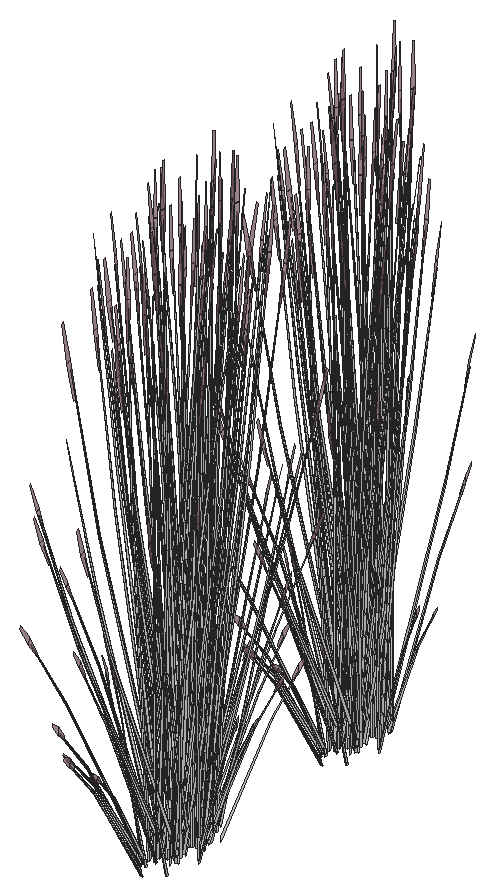
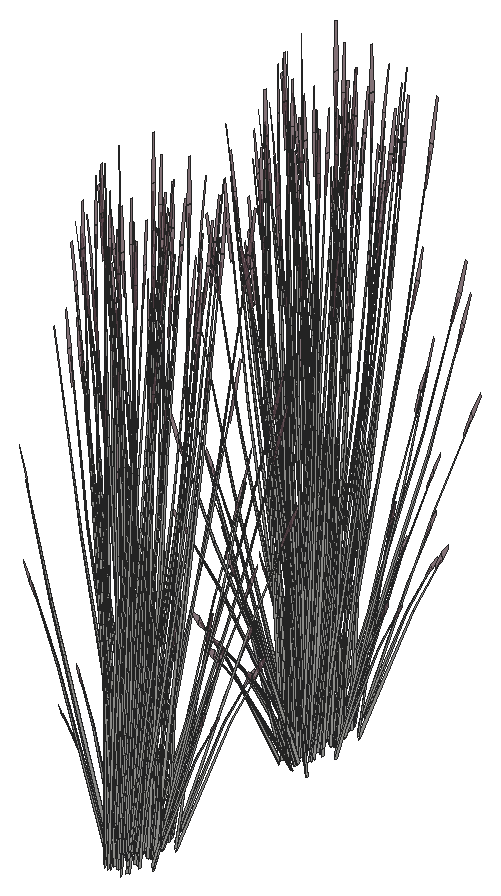
# SketchUp Ruby script. Lengths in inches.
U = 1.inch
M = Sketchup.active_model
def pt(a) = Geom::Point3d.new(a.map { |v| v * U })
def face(e, loops, mat)
  f = e.add_face(loops[0].map { |a| pt(a) })
  loops[1..].each { |l| e.add_face(l.map { |a| pt(a) }).erase! }
  f.material = f.back_material = mat if mat
  f
end
# faces: each face lists its corners as indices into pts; further lists are holes
def faces(e, pts, list, mat = nil) = list.each { |f| face(e, (f[0].is_a?(Array) ? f : [f]).map { |l| l.map { |i| pts[i] } }, mat) }
# xy, xz, yz: faces in a plane at the given z, y or x. An outline is a flat list of corners, or four numbers for a rectangle; further outlines are holes
def ring(l) = l.size == 4 ? [[l[0], l[1]], [l[2], l[1]], [l[2], l[3]], [l[0], l[3]]] : l.each_slice(2).to_a
def flat(e, list, mat, &to3) = list.each { |f| face(e, (f[0].is_a?(Array) ? f : [f]).map { |l| ring(l).map { |u, v| to3.(u, v) } }, mat) }
def xy(e, z, list, mat = nil) = flat(e, list, mat) { |x, y| [x, y, z] }
def xz(e, y, list, mat = nil) = flat(e, list, mat) { |x, z| [x, y, z] }
def yz(e, x, list, mat = nil) = flat(e, list, mat) { |y, z| [x, y, z] }
def lines(e, pts, list) = list.each { |a, b| e.add_line(pt(pts[a]), pt(pts[b])) }
# prism: a flat outline (further loops are holes) pulled along v
def prism(e, loops, v, mat = nil)
  f = face(e, loops, mat); d = Geom::Vector3d.new(v.map { |x| x * U })
  f.pushpull(f.normal.samedirection?(d) ? d.length : -d.length)
end
def box(e, o, s, mat = nil) = prism(e, [[o, [o[0] + s[0], o[1], o[2]], [o[0] + s[0], o[1] + s[1], o[2]], [o[0], o[1] + s[1], o[2]]]], [0, 0, s[2]], mat)
def at(x, y, z, deg = 0) = Geom::Transformation.translation(pt([x, y, z])) * Geom::Transformation.rotation(ORIGIN, Z_AXIS, deg.degrees)
def axes(o, x, y, z) = Geom::Transformation.new([*x, 0, *y, 0, *z, 0, *pt(o).to_a, 1])
def part(name) = M.definitions.add(name)
# library, detail: a bought-in or finely detailed component or shape, given as its bounding box
def library(name, o, s) = part(name).tap { |d| box(d.entities, o, s) }
def detail(e, o, s) = box(e.add_group.entities, o, s)
def put(e, d, t, mat = nil) = e.add_instance(d, t).tap { |i| i.material = mat if mat }
def group(e, t, mat = nil) = e.add_group.tap { |g| g.transformation = t; g.material = mat if mat }.entities
root = M.entities
M.materials.add("LightPink_Translucent").color = [144, 107, 117]
M.materials["LightPink_Translucent"].alpha = 0.75
c1 = part("blade")
p = [[2.15,0.21,22],[0,0.17,0],[0.09,0.45,0],[2.18,0.31,22],[2.29,0.31,22],[0.38,0.45,0],
  [2.48,0.24,33],[2.49,0.24,33],[2.48,0.22,33]]
faces(c1.entities,p,[[0,1,2,3],[4,5,2,3],[6,3,4,7],[8,0,3,6]])
c2 = part("seeds")
p = [[0.3,-0.1,1.38],[-0.01,-0.03,1.59],[-0.01,-0.03,0.03],[0.14,-0.07,-0.07],[0.29,-0.03,3],[0.15,0.01,3.11]]
faces(c2.entities,p,[[0,1,2,3],[1,0,4,5]],"LightPink_Translucent")
c3 = part("blade with seeds")
put(c3.entities,c1,at(0,0,0))
put(c3.entities,c2,axes([2.4,0.25,30.99],[1.5799,-0.05474,1.17369],[-0.12525,1.92788,0.29478],[-0.07173,-0.02425,1.56792]))
put(root,c3,axes([252.15,10.32,1.07],[-0.07276,0.12376,1.03788],[-0.21789,-0.21662,-0.22321],[0.04039,-0.2694,0.44375]))
put(root,c3,axes([251.82,10.75,2.81],[-0.12216,-0.49718,-0.51563],[0.25147,-0.27708,0.06223],[-0.02857,-0.24022,0.72942]))
put(root,c3,axes([251.03,10.09,1.07],[-0.0155,0.20002,1.03788],[-0.22659,0.16744,-0.22321],[-0.05297,-0.25854,0.44375]))
put(root,c3,axes([251.61,9.65,0.28],[-0.04293,0.02203,1.27986],[-0.23742,-0.24798,-0.19552],[0.00398,-0.20684,0.218]))
put(root,c3,axes([252.33,11.24,2.81],[0.00666,-0.56559,-0.51563],[0.28045,0.03799,0.06223],[0.0296,-0.23961,0.72942]))
put(root,c3,axes([251.88,9.33,1.2],[0.03283,0.35655,0.83364],[-0.18215,-0.19748,0.6125],[0.0196,-0.18257,0.18362]))
put(root,c3,axes([250.95,9.76,1.2],[0.13352,0.21281,0.83364],[-0.19445,0.12793,0.6125],[-0.0416,-0.16355,0.18362]))
put(root,c3,axes([251.27,10.89,2.81],[-0.21825,-0.29555,-0.51563],[0.15511,-0.5179,0.06223],[-0.07907,-0.17646,0.72942]))
put(root,c3,axes([250.84,10.4,0.28],[-0.02479,0.08055,1.27986],[-0.25056,0.17367,-0.19552],[-0.06053,-0.15798,0.218]))
put(root,c3,axes([251.25,12.62,0.72],[-0.10512,-0.62701,-0.50685],[0.30279,-0.22582,-0.13303],[-0.01162,-0.21232,1.11879]))
put(root,c3,axes([252.66,10.7,0.28],[-0.03831,-0.04817,1.27986],[-0.0984,-0.53815,-0.19552],[0.06638,-0.14604,0.218]))
put(root,c3,axes([252.66,12.22,2.81],[0.1337,-0.48245,-0.51563],[0.23429,0.34287,0.06223],[0.07983,-0.1748,0.72942]))
put(root,c3,axes([251.21,10.81,0.91],[-0.16003,-0.61271,0],[0.26773,-0.34169,-0.37456],[0.06098,-0.07782,1.18819]))
put(root,c3,axes([251.56,10.08,0.74],[-0.17688,0.35078,-0.02825],[-0.16207,-0.38418,-0.1281],[-0.01141,-0.10886,0.42251]))
put(root,c3,axes([250.64,12.53,0.66],[0,-0.61145,-0.36036],[0.28637,0,0],[0,-0.13926,1.14313]))
put(root,c3,axes([251.43,10.72,0.66],[0.23955,-0.30573,-0.36036],[0.14318,0.54821,0],[0.05456,-0.06963,1.14313]))
put(root,c3,axes([252.85,11.78,1.07],[-0.09144,-0.01811,1.03788],[-0.09368,-0.48584,-0.22321],[0.11233,-0.13744,0.44375]))
put(root,c3,axes([251.71,11.97,0.6875],[0.1724,-0.45959,-0.45255],[0.21416,0.41674,-0.11877],[0.06908,-0.11465,0.99892]))
put(root,c3,axes([252.96,10.88,1.2],[-0.08525,0.31126,0.83364],[-0.07328,-0.41819,0.6125],[0.07041,-0.10479,0.18362]))
put(root,c3,axes([251.41,12.78,0.8],[0.12419,-0.55096,-0.32471],[0.25804,0.26516,0.15627],[0,-0.12701,1.04254]))
put(root,c3,axes([251.53,12.51,1.13],[-0.02983,-0.6977,-0.21117],[0.31064,-0.04219,-0.36291],[0.0547,-0.09294,1.15913]))
put(root,c3,axes([250.76,12.54,0.66],[0.17867,-0.3815,-0.22483],[0.17867,0.3815,0.22483],[0,-0.12288,1.00865]))
put(root,c3,axes([250.6875,10.71,0.74],[-0.07384,0.49928,-0.02825],[-0.22725,-0.15358,-0.1281],[-0.0345,-0.08166,0.42251]))
put(root,c3,axes([251.38,13.24,1.13],[-0.28825,-0.29175,-0.21117],[0.1388,-0.61578,-0.36291],[-0.00906,-0.15119,1.15913]))
put(root,c3,axes([250.5625,12.99,0.91],[-0.32006,0,0],[0,-0.68339,-0.37456],[0,-0.15565,1.18819]))
put(root,c3,axes([250.62,11.77,1.07],[0.04997,0.17024,1.03788],[-0.11515,0.46273,-0.22321],[-0.11824,-0.1106,0.44375]))
put(root,c3,axes([251.49,10.96,0.66],[0.23879,0.15129,-0.22483],[-0.06012,0.53279,0.22483],[0.04814,-0.06144,1.00865]))
put(root,c3,axes([250.82,11.62,2.81],[-0.25586,-0.01472,-0.51563],[0.01718,-0.61995,0.06223],[-0.1084,-0.06542,0.72942]))
put(root,c3,axes([250.8125,12.8125,0.88],[-0.23808,0.51407,0.22322],[-0.23822,-0.50866,-0.26485],[-0.00831,-0.14599,1.19671]))
put(root,c3,axes([251.57,13.05,0.96],[0.28839,0.29636,0.17466],[-0.1388,0.61578,0.36291],[0,-0.14195,1.16519]))
put(root,c3,axes([251.46,13.89,0.96],[0.06784,-0.72454,-0.17004],[0.32166,0.1263,0.37211],[-0.05621,-0.10006,1.13542]))
put(root,c3,axes([250.32,12.28,1.2],[0.16341,-0.04375,0.83364],[-0.10366,0.38551,0.6125],[-0.08075,-0.05783,0.18362]))
put(root,c3,axes([251.48,12.64,1.17],[-0.27795,0.03775,0.32471],[-0.02514,-0.62656,-0.15627],[0.04976,-0.0635,1.04254]))
put(root,c3,axes([250.76,13.1,0.99],[0,0.61145,0.36036],[-0.28637,0,0],[0,-0.13926,1.14313]))
put(root,c3,axes([252.39,10.97,0.92],[0.16003,-0.61271,0],[0.26773,0.34169,-0.37456],[0.06098,0.07782,1.18819]))
put(root,c3,axes([251.43,13.59,0.8],[-0.15376,-0.51322,-0.32471],[0.2329,-0.3614,0.15627],[-0.04976,-0.0635,1.04254]))
put(root,c3,axes([251.47,12.87,0.91],[0.11128,0.68373,0.33208],[-0.31797,0.23776,0.13031],[0.00389,-0.12563,1.15295]))
put(root,c3,axes([253.02,13.39,0.63],[-0.16485,0.07338,1.02759],[-0.02624,-0.58408,0.05882],[0.11546,-0.08841,0.58473]))
put(root,c3,axes([253.32,12.875,0.83],[-0.15869,-0.39099,-0.04709],[0.1738,-0.35825,-0.21349],[0.04925,-0.02522,0.70419]))
put(root,c3,axes([251.41,13.4,1.17],[-0.12419,0.55096,0.32471],[-0.25804,-0.26516,-0.15627],[0,-0.12701,1.04254]))
put(root,c3,axes([251.87,12.92,0.79],[0,-0.70749,0],[0.32006,0,0],[0,0,1.30246]))
put(root,c3,axes([252.25,11.29,0.99],[-0.23955,-0.30573,0.36036],[0.14318,-0.54821,0],[0.05456,0.06963,1.14313]))
put(root,c3,axes([252.72,13.4375,2.81],[0.22491,-0.27005,-0.51563],[0.12534,0.55588,0.06223],[0.10867,-0.06315,0.72942]))
put(root,c3,axes([251.3,13.79,0.6875],[-0.26625,-0.10025,-0.45255],[0.05619,-0.61836,-0.11877],[-0.07946,-0.07493,0.99892]))
put(root,c3,axes([251.71,12.48,0.91],[-0.21222,0.5549,0.33208],[-0.25213,-0.48983,0.13031],[0.05116,-0.05538,1.15295]))
put(root,c3,axes([251.95,13.47,0.86],[-0.23808,-0.52628,-0.0445],[0.23822,-0.5266,0],[-0.00831,-0.01838,1.27426]))
put(root,c3,axes([251.35,11.56,0.99],[-0.07394,0.60768,0.12804],[-0.27057,-0.17197,0.25465],[0.04674,-0.00296,1.1642]))
put(root,c3,axes([251.23,12.06,0.35],[-0.25194,0.2448,0.93574],[-0.08019,-0.7024,0.36359],[0.1547,0.01169,1.0643]))
put(root,c3,axes([251.91,12.24,1.09],[0.04938,-0.54569,0.10509],[0.24125,0.09472,-0.30009],[0.0439,0.05603,0.91989]))
put(root,c3,axes([251.49,13.54,0.91],[0.32351,0.12883,0.33208],[-0.06584,0.72759,0.13031],[-0.04728,-0.07026,1.15295]))
put(root,c3,axes([253.2,13.01,0.28],[-0.01338,-0.09283,1.27986],[0.09278,-0.54301,-0.19552],[0.09359,-0.00781,0.218]))
put(root,c3,axes([250.44,12.91,0.28],[0.00649,0.09636,1.27986],[-0.13086,0.50324,-0.19552],[-0.09295,-0.02537,0.218]))
put(root,c3,axes([251.81,12.38,1.17],[-0.15376,-0.51322,0.32471],[0.2329,-0.3614,-0.15627],[0.04976,0.0635,1.04254]))
put(root,c3,axes([251.01,14.73,0.66],[-0.06012,-0.53279,-0.22483],[0.23879,-0.15129,0.22483],[-0.04814,-0.06144,1.00865]))
put(root,c3,axes([251.32,14.7,0.99],[0.27504,-0.16229,0.12804],[0.06792,0.60396,0.25465],[-0.02453,-0.088,1.1642]))
put(root,c3,axes([251.89,12.42,1.13],[0.25843,-0.40595,-0.21117],[0.17185,0.5736,-0.36291],[0.06376,0.05825,1.15913]))
put(root,c3,axes([250.95,14.96,0.66],[-0.23955,-0.30573,-0.36036],[0.14318,-0.54821,0],[-0.05456,-0.06963,1.14313]))
put(root,c3,axes([252.54,11.34,0.66],[0.23955,0.30573,-0.36036],[-0.14318,0.54821,0],[0.05456,0.06963,1.14313]))
put(root,c3,axes([252.08,13.08,0.79],[0.28637,0,0],[0,0.63302,0],[0,0,1.29484]))
put(root,c3,axes([251.6,13.88,1.13],[-0.25843,0.40595,-0.21117],[-0.17185,-0.5736,-0.36291],[-0.06376,-0.05825,1.15913]))
put(root,c3,axes([252.16,11.6,0.99],[-0.27504,0.16229,0.12804],[-0.06792,-0.60396,0.25465],[0.02453,0.088,1.1642]))
put(root,c3,axes([252.47,11.57,0.66],[0.06012,0.53279,-0.22483],[-0.23879,0.15129,0.22483],[0.04814,0.06144,1.00865]))
put(root,c3,axes([251.99,12.76,0.92],[-0.32351,-0.12883,0.35707],[0.06584,-0.72759,0.14012],[0.04728,0.07026,1.23973]))
put(root,c3,axes([251.73,14.56,0.79],[-0.08351,-0.52716,0],[0.23848,-0.18461,0],[0,0,1.1204]))
put(root,c3,axes([251.57,14.06,1.09],[-0.04938,0.54569,0.10509],[-0.24125,-0.09472,-0.30009],[-0.0439,-0.05603,0.91989]))
put(root,c3,axes([252.05,14.48,0.78],[0.26872,-0.20746,-0.13933],[0.09442,0.59762,0.00006],[0.02966,-0.02293,1.26212]))
put(root,c3,axes([252.14,14.73,0.99],[0.07394,-0.60768,0.12804],[0.27057,0.17197,0.25465],[-0.04674,0.00296,1.1642]))
put(root,c3,axes([252.08,13.35,0.8],[0.17867,0.39495,0],[-0.17867,0.39495,0],[0,0,1.22851]))
put(root,c3,axes([252.5625,13.18,0.99],[-0.2011,-0.44539,0.12804],[0.20266,-0.432,0.25465],[-0.02221,0.09096,1.1642]))
put(root,c3,axes([252.1875,12.51,0.6875],[0.26625,0.10025,-0.45255],[-0.05619,0.61836,-0.11877],[0.07946,0.07493,0.99892]))
put(root,c3,axes([253.36,13.59,1.2],[-0.15814,0.10094,0.83364],[0.07444,-0.41719,0.6125],[0.0839,0.02855,0.18362]))
put(root,c3,axes([251.67,14.79,0.79],[-0.25804,-0.27452,0],[0.12419,-0.5704,0],[0,0,1.1809]))
put(root,c3,axes([251.89,14.0625,0.98],[-0.24993,-0.49214,-0.18284],[0.21031,-0.55263,0.40012],[-0.0673,0.05757,1.22088]))
put(root,c3,axes([251.23,15.01,0.99],[0.23955,0.30573,0.36036],[-0.14318,0.54821,0],[-0.05456,-0.06963,1.14313]))
put(root,c3,axes([252.07,12.89,1.17],[0.12419,-0.55096,0.32471],[0.25804,0.26516,-0.15627],[0,0.12701,1.04254]))
put(root,c3,axes([252.03,13.21,0.86],[0,0.70714,-0.04091],[-0.32006,0,0],[0,0.02222,1.30182]))
put(root,c3,axes([252.05,12.71,0.8],[0.15376,0.51322,-0.32471],[-0.2329,0.3614,0.15627],[0.04976,0.0635,1.04254]))
put(root,c3,axes([251.09,15.33,0.91],[-0.16003,0.61271,0],[-0.26773,-0.34169,-0.37456],[-0.06098,-0.07782,1.18819]))
put(root,c3,axes([252.73,13.2,0.99],[0,-0.61145,0.36036],[0.28637,0,0],[0,0.13926,1.14313]))
put(root,c3,axes([252.01,13.66,1.17],[0.27795,-0.03775,0.32471],[0.02514,0.62656,-0.15627],[-0.04976,0.0635,1.04254]))
put(root,c3,axes([252.18,13.02,1.09],[0.23848,-0.17832,0.10509],[0.08351,0.5092,-0.30009],[0,0.11207,0.91989]))
put(root,c3,axes([251.76,13.96,0.8],[-0.27795,0.03775,-0.32471],[-0.02514,-0.62656,0.15627],[-0.04976,0.0635,1.04254]))
put(root,c3,axes([253.07,14.26,1.07],[-0.06164,-0.15038,1.03788],[0.0802,-0.49748,-0.22321],[0.12472,0.06739,0.44375]))
put(root,c3,axes([251.97,14.81,0.79],[0.25804,0.27452,0],[-0.12419,0.5704,0],[0,0,1.26978]))
put(root,c3,axes([252.07,15.41,0.78],[-0.15803,-0.61485,-0.03732],[0.26773,-0.34169,0.37456],[-0.06597,0.05854,1.1876]))
put(root,c3,axes([252.01,13.93,1.09],[0.1891,0.36737,0.10509],[-0.15773,0.41447,-0.30009],[-0.0439,0.05603,0.91989]))
put(root,c3,axes([252.5,14.5625,2.81],[0.25586,0.01472,-0.51563],[-0.01718,0.61995,0.06223],[0.1084,0.06542,0.72942]))
put(root,c3,axes([252.21,15.06,0.99],[0.23955,-0.30573,0.36036],[0.14318,0.54821,0],[-0.05456,0.06963,1.14313]))
put(root,c3,axes([251.875,14.57,0.86],[0.11128,0.70245,-0.04364],[-0.31797,0.24614,0],[0.00389,0.02453,1.2496]))
put(root,c3,axes([252,15.33,0.66],[-0.23879,-0.15129,-0.22483],[0.06012,-0.53279,0.22483],[-0.04814,0.06144,1.00865]))
put(root,c3,axes([250.27,14.25,1.07],[0.08895,0.05019,1.03788],[0.05733,0.5127,-0.22321],[-0.12083,0.09597,0.44375]))
put(root,c3,axes([252.92,13.3,0.92],[0.32006,0,0],[0,0.68339,-0.37456],[0,0.15565,1.18819]))
put(root,c3,axes([252.79,13.65,0.79],[-0.3199,-0.00489,-0.03612],[0,-0.68339,0.36248],[-0.01005,0.15557,1.14929]))
put(root,c3,axes([252.1,13.06,1.13],[0.28825,0.29175,-0.21117],[-0.1388,0.61578,-0.36291],[0.00906,0.15119,1.15913]))
put(root,c3,axes([250.09,15.33,1.2],[0.10667,-0.27712,0.83364],[0.04209,0.43871,0.6125],[-0.07709,0.07855,0.18362]))
put(root,c3,axes([252.73,13.75,0.66],[-0.17867,0.3815,-0.22483],[-0.17867,-0.3815,0.22483],[0,0.12288,1.00865]))
put(root,c3,axes([251.96,13.79,1.13],[0.02983,0.6977,-0.21117],[-0.31064,0.04219,-0.36291],[-0.0547,0.09294,1.15913]))
put(root,c3,axes([252.07,13.52,0.8],[-0.12419,0.55096,-0.32471],[-0.25804,-0.26516,0.15627],[0,0.12701,1.04254]))
put(root,c3,axes([251.77,14.32,0.6875],[-0.1724,0.45959,-0.45255],[-0.21416,-0.41674,-0.11877],[-0.06908,0.11465,0.99892]))
put(root,c3,axes([252.08,15.1,0.88],[0.32044,0.19874,0.22322],[-0.08017,0.71038,-0.26485],[-0.05304,0.08891,1.19671]))
put(root,c3,axes([252.05,15.58,0.66],[-0.23955,0.30573,-0.36036],[-0.14318,-0.54821,0],[-0.05456,0.06963,1.14313]))
put(root,c3,axes([252.85,13.77,0.66],[0,0.61145,-0.36036],[-0.28637,0,0],[0,0.13926,1.14313]))
put(root,c3,axes([252.49,15.03,1.2],[-0.14411,-0.17581,0.83364],[0.18609,-0.17864,0.6125],[0.05019,0.15132,0.18362]))
put(root,c3,axes([252.27,15.48,0.91],[0.16003,0.61271,0],[-0.26773,0.34169,-0.37456],[-0.06098,0.07782,1.18819]))
put(root,c3,axes([252.53,15.6875,0.28],[0.01865,-0.08828,1.27986],[0.23477,-0.25998,-0.19552],[0.07118,0.13456,0.218]))
put(root,c3,axes([252.13,13.06,1.26],[-0.00699,-0.5757,1.02533],[0.31645,0.14923,0.43413],[-0.07484,0.31502,0.96783]))
put(root,c3,axes([252.22,13.68,0.71],[0.09385,0.55983,-0.50233],[-0.27035,0.20162,-0.13184],[0.01037,0.18957,1.1088]))
put(root,c3,axes([250.37,15.61,0.28],[0.03433,0.06109,1.27986],[0.05822,0.56601,-0.19552],[-0.07609,0.1207,0.218]))
put(root,c3,axes([252.51,15.84,1.13],[-0.16414,-0.01918,0.76251],[0.10839,-0.40729,0.421],[0.06484,0.1447,0.59812]))
put(root,c3,axes([251.97,14.85,1.07],[0.00452,-0.20269,1.03788],[0.21585,-0.22641,-0.22321],[0.06663,0.2426,0.44375]))
put(root,c3,axes([250.99,16.54,1.2],[-0.00662,-0.36357,0.83364],[0.16552,0.25931,0.6125],[-0.03255,0.17329,0.18362]))
put(root,c3,axes([251.43,15.67,0.28],[0.04142,-0.03327,1.27986],[0.24917,0.18313,-0.19552],[0.00729,0.2064,0.218]))
put(root,c3,axes([250.86,15.75,1.24],[0.23252,-0.10828,0.04723],[0.05346,0.43623,-0.62638],[-0.01474,0.22082,0.56147]))
put(root,c3,axes([251.51,15.43,2.81],[0.12216,0.49718,-0.51563],[-0.25147,0.27708,0.06223],[0.02857,0.24022,0.72942]))
put(root,c3,axes([250.8,16.21,1.07],[0.08077,-0.09646,1.03788],[0.19942,0.29084,-0.22321],[-0.05936,0.25166,0.44375]))
put(root,c3,axes([252.15,27.1875,1.07],[-0.07276,0.12376,1.03788],[-0.21789,-0.21662,-0.22321],[0.04039,-0.2694,0.44375]))
put(root,c3,axes([251.82,27.62,2.81],[-0.12216,-0.49718,-0.51563],[0.25147,-0.27708,0.06223],[-0.02857,-0.24022,0.72942]))
put(root,c3,axes([251.03,26.95,1.07],[-0.0155,0.20002,1.03788],[-0.22659,0.16744,-0.22321],[-0.05297,-0.25854,0.44375]))
put(root,c3,axes([251.61,26.52,0.28],[-0.04293,0.02203,1.27986],[-0.23742,-0.24798,-0.19552],[0.00398,-0.20684,0.218]))
put(root,c3,axes([252.33,28.1,2.81],[0.00666,-0.56559,-0.51563],[0.28045,0.03799,0.06223],[0.0296,-0.23961,0.72942]))
put(root,c3,axes([251.88,26.2,1.2],[0.03283,0.35655,0.83364],[-0.18215,-0.19748,0.6125],[0.0196,-0.18257,0.18362]))
put(root,c3,axes([250.95,26.63,1.2],[0.13352,0.21281,0.83364],[-0.19445,0.12793,0.6125],[-0.0416,-0.16355,0.18362]))
put(root,c3,axes([251.27,27.76,2.81],[-0.21825,-0.29555,-0.51563],[0.15511,-0.5179,0.06223],[-0.07907,-0.17646,0.72942]))
put(root,c3,axes([250.84,27.27,0.28],[-0.02479,0.08055,1.27986],[-0.25056,0.17367,-0.19552],[-0.06053,-0.15798,0.218]))
put(root,c3,axes([251.25,29.49,0.72],[-0.10512,-0.62701,-0.50685],[0.30279,-0.22582,-0.13303],[-0.01162,-0.21232,1.11879]))
put(root,c3,axes([252.66,27.57,0.28],[-0.03831,-0.04817,1.27986],[-0.0984,-0.53815,-0.19552],[0.06638,-0.14604,0.218]))
put(root,c3,axes([252.66,29.09,2.81],[0.1337,-0.48245,-0.51563],[0.23429,0.34287,0.06223],[0.07983,-0.1748,0.72942]))
put(root,c3,axes([251.21,27.68,0.91],[-0.16003,-0.61271,0],[0.26773,-0.34169,-0.37456],[0.06098,-0.07782,1.18819]))
put(root,c3,axes([251.56,26.95,0.74],[-0.17688,0.35078,-0.02825],[-0.16207,-0.38418,-0.1281],[-0.01141,-0.10886,0.42251]))
put(root,c3,axes([250.64,29.4,0.66],[0,-0.61145,-0.36036],[0.28637,0,0],[0,-0.13926,1.14313]))
put(root,c3,axes([251.43,27.59,0.66],[0.23955,-0.30573,-0.36036],[0.14318,0.54821,0],[0.05456,-0.06963,1.14313]))
put(root,c3,axes([252.85,28.64,1.07],[-0.09144,-0.01811,1.03788],[-0.09368,-0.48584,-0.22321],[0.11233,-0.13744,0.44375]))
put(root,c3,axes([251.71,28.84,0.6875],[0.1724,-0.45959,-0.45255],[0.21416,0.41674,-0.11877],[0.06908,-0.11465,0.99892]))
put(root,c3,axes([252.96,27.75,1.2],[-0.08525,0.31126,0.83364],[-0.07328,-0.41819,0.6125],[0.07041,-0.10479,0.18362]))
put(root,c3,axes([251.41,29.65,0.8],[0.12419,-0.55096,-0.32471],[0.25804,0.26516,0.15627],[0,-0.12701,1.04254]))
put(root,c3,axes([251.53,29.375,1.13],[-0.02983,-0.6977,-0.21117],[0.31064,-0.04219,-0.36291],[0.0547,-0.09294,1.15913]))
put(root,c3,axes([250.76,29.41,0.66],[0.17867,-0.3815,-0.22483],[0.17867,0.3815,0.22483],[0,-0.12288,1.00865]))
put(root,c3,axes([250.6875,27.58,0.74],[-0.07384,0.49928,-0.02825],[-0.22725,-0.15358,-0.1281],[-0.0345,-0.08166,0.42251]))
put(root,c3,axes([251.38,30.11,1.13],[-0.28825,-0.29175,-0.21117],[0.1388,-0.61578,-0.36291],[-0.00906,-0.15119,1.15913]))
put(root,c3,axes([250.5625,29.86,0.91],[-0.32006,0,0],[0,-0.68339,-0.37456],[0,-0.15565,1.18819]))
put(root,c3,axes([250.62,28.64,1.07],[0.04997,0.17024,1.03788],[-0.11515,0.46273,-0.22321],[-0.11824,-0.1106,0.44375]))
put(root,c3,axes([251.49,27.83,0.66],[0.23879,0.15129,-0.22483],[-0.06012,0.53279,0.22483],[0.04814,-0.06144,1.00865]))
put(root,c3,axes([250.82,28.49,2.81],[-0.25586,-0.01472,-0.51563],[0.01718,-0.61995,0.06223],[-0.1084,-0.06542,0.72942]))
put(root,c3,axes([250.8125,29.68,0.88],[-0.23808,0.51407,0.22322],[-0.23822,-0.50866,-0.26485],[-0.00831,-0.14599,1.19671]))
put(root,c3,axes([251.57,29.92,0.96],[0.28839,0.29636,0.17466],[-0.1388,0.61578,0.36291],[0,-0.14195,1.16519]))
put(root,c3,axes([251.46,30.75,0.96],[0.06784,-0.72454,-0.17004],[0.32166,0.1263,0.37211],[-0.05621,-0.10006,1.13542]))
put(root,c3,axes([250.32,29.15,1.2],[0.16341,-0.04375,0.83364],[-0.10366,0.38551,0.6125],[-0.08075,-0.05783,0.18362]))
put(root,c3,axes([251.48,29.51,1.17],[-0.27795,0.03775,0.32471],[-0.02514,-0.62656,-0.15627],[0.04976,-0.0635,1.04254]))
put(root,c3,axes([250.76,29.97,0.99],[0,0.61145,0.36036],[-0.28637,0,0],[0,-0.13926,1.14313]))
put(root,c3,axes([252.39,27.84,0.92],[0.16003,-0.61271,0],[0.26773,0.34169,-0.37456],[0.06098,0.07782,1.18819]))
put(root,c3,axes([251.43,30.46,0.8],[-0.15376,-0.51322,-0.32471],[0.2329,-0.3614,0.15627],[-0.04976,-0.0635,1.04254]))
put(root,c3,axes([251.47,29.73,0.91],[0.11128,0.68373,0.33208],[-0.31797,0.23776,0.13031],[0.00389,-0.12563,1.15295]))
put(root,c3,axes([253.02,30.26,0.63],[-0.16485,0.07338,1.02759],[-0.02624,-0.58408,0.05882],[0.11546,-0.08841,0.58473]))
put(root,c3,axes([253.32,29.74,0.83],[-0.15869,-0.39099,-0.04709],[0.1738,-0.35825,-0.21349],[0.04925,-0.02522,0.70419]))
put(root,c3,axes([251.41,30.27,1.17],[-0.12419,0.55096,0.32471],[-0.25804,-0.26516,-0.15627],[0,-0.12701,1.04254]))
put(root,c3,axes([251.87,29.79,0.79],[0,-0.70749,0],[0.32006,0,0],[0,0,1.30246]))
put(root,c3,axes([252.25,28.16,0.99],[-0.23955,-0.30573,0.36036],[0.14318,-0.54821,0],[0.05456,0.06963,1.14313]))
put(root,c3,axes([252.72,30.3,2.81],[0.22491,-0.27005,-0.51563],[0.12534,0.55588,0.06223],[0.10867,-0.06315,0.72942]))
put(root,c3,axes([251.3,30.66,0.6875],[-0.26625,-0.10025,-0.45255],[0.05619,-0.61836,-0.11877],[-0.07946,-0.07493,0.99892]))
put(root,c3,axes([251.71,29.35,0.91],[-0.21222,0.5549,0.33208],[-0.25213,-0.48983,0.13031],[0.05116,-0.05538,1.15295]))
put(root,c3,axes([251.95,30.34,0.86],[-0.23808,-0.52628,-0.0445],[0.23822,-0.5266,0],[-0.00831,-0.01838,1.27426]))
put(root,c3,axes([251.35,28.43,0.99],[-0.07394,0.60768,0.12804],[-0.27057,-0.17197,0.25465],[0.04674,-0.00296,1.1642]))
put(root,c3,axes([251.23,28.92,0.35],[-0.25194,0.2448,0.93574],[-0.08019,-0.7024,0.36359],[0.1547,0.01169,1.0643]))
put(root,c3,axes([251.91,29.11,1.09],[0.04938,-0.54569,0.10509],[0.24125,0.09472,-0.30009],[0.0439,0.05603,0.91989]))
put(root,c3,axes([251.49,30.4,0.91],[0.32351,0.12883,0.33208],[-0.06584,0.72759,0.13031],[-0.04728,-0.07026,1.15295]))
put(root,c3,axes([253.2,29.88,0.28],[-0.01338,-0.09283,1.27986],[0.09278,-0.54301,-0.19552],[0.09359,-0.00781,0.218]))
put(root,c3,axes([250.44,29.78,0.28],[0.00649,0.09636,1.27986],[-0.13086,0.50324,-0.19552],[-0.09295,-0.02537,0.218]))
put(root,c3,axes([251.81,29.25,1.17],[-0.15376,-0.51322,0.32471],[0.2329,-0.3614,-0.15627],[0.04976,0.0635,1.04254]))
put(root,c3,axes([251.01,31.6,0.66],[-0.06012,-0.53279,-0.22483],[0.23879,-0.15129,0.22483],[-0.04814,-0.06144,1.00865]))
put(root,c3,axes([251.32,31.57,0.99],[0.27504,-0.16229,0.12804],[0.06792,0.60396,0.25465],[-0.02453,-0.088,1.1642]))
put(root,c3,axes([251.89,29.29,1.13],[0.25843,-0.40595,-0.21117],[0.17185,0.5736,-0.36291],[0.06376,0.05825,1.15913]))
put(root,c3,axes([250.95,31.83,0.66],[-0.23955,-0.30573,-0.36036],[0.14318,-0.54821,0],[-0.05456,-0.06963,1.14313]))
put(root,c3,axes([252.54,28.21,0.66],[0.23955,0.30573,-0.36036],[-0.14318,0.54821,0],[0.05456,0.06963,1.14313]))
put(root,c3,axes([252.08,29.95,0.79],[0.28637,0,0],[0,0.63302,0],[0,0,1.29484]))
put(root,c3,axes([251.6,30.75,1.13],[-0.25843,0.40595,-0.21117],[-0.17185,-0.5736,-0.36291],[-0.06376,-0.05825,1.15913]))
put(root,c3,axes([252.16,28.47,0.99],[-0.27504,0.16229,0.12804],[-0.06792,-0.60396,0.25465],[0.02453,0.088,1.1642]))
put(root,c3,axes([252.47,28.43,0.66],[0.06012,0.53279,-0.22483],[-0.23879,0.15129,0.22483],[0.04814,0.06144,1.00865]))
put(root,c3,axes([251.99,29.63,0.92],[-0.32351,-0.12883,0.35707],[0.06584,-0.72759,0.14012],[0.04728,0.07026,1.23973]))
put(root,c3,axes([251.73,31.42,0.79],[-0.08351,-0.52716,0],[0.23848,-0.18461,0],[0,0,1.1204]))
put(root,c3,axes([251.57,30.92,1.09],[-0.04938,0.54569,0.10509],[-0.24125,-0.09472,-0.30009],[-0.0439,-0.05603,0.91989]))
put(root,c3,axes([252.05,31.35,0.78],[0.26872,-0.20746,-0.13933],[0.09442,0.59762,0.00006],[0.02966,-0.02293,1.26212]))
put(root,c3,axes([252.14,31.6,0.99],[0.07394,-0.60768,0.12804],[0.27057,0.17197,0.25465],[-0.04674,0.00296,1.1642]))
put(root,c3,axes([252.08,30.22,0.8],[0.17867,0.39495,0],[-0.17867,0.39495,0],[0,0,1.22851]))
put(root,c3,axes([252.5625,30.05,0.99],[-0.2011,-0.44539,0.12804],[0.20266,-0.432,0.25465],[-0.02221,0.09096,1.1642]))
put(root,c3,axes([252.1875,29.38,0.6875],[0.26625,0.10025,-0.45255],[-0.05619,0.61836,-0.11877],[0.07946,0.07493,0.99892]))
put(root,c3,axes([253.36,30.46,1.2],[-0.15814,0.10094,0.83364],[0.07444,-0.41719,0.6125],[0.0839,0.02855,0.18362]))
put(root,c3,axes([251.67,31.66,0.79],[-0.25804,-0.27452,0],[0.12419,-0.5704,0],[0,0,1.1809]))
put(root,c3,axes([251.89,30.93,0.98],[-0.24993,-0.49214,-0.18284],[0.21031,-0.55263,0.40012],[-0.0673,0.05757,1.22088]))
put(root,c3,axes([251.23,31.875,0.99],[0.23955,0.30573,0.36036],[-0.14318,0.54821,0],[-0.05456,-0.06963,1.14313]))
put(root,c3,axes([252.07,29.76,1.17],[0.12419,-0.55096,0.32471],[0.25804,0.26516,-0.15627],[0,0.12701,1.04254]))
put(root,c3,axes([252.03,30.07,0.86],[0,0.70714,-0.04091],[-0.32006,0,0],[0,0.02222,1.30182]))
put(root,c3,axes([252.05,29.57,0.8],[0.15376,0.51322,-0.32471],[-0.2329,0.3614,0.15627],[0.04976,0.0635,1.04254]))
put(root,c3,axes([251.09,32.2,0.91],[-0.16003,0.61271,0],[-0.26773,-0.34169,-0.37456],[-0.06098,-0.07782,1.18819]))
put(root,c3,axes([252.73,30.07,0.99],[0,-0.61145,0.36036],[0.28637,0,0],[0,0.13926,1.14313]))
put(root,c3,axes([252.01,30.52,1.17],[0.27795,-0.03775,0.32471],[0.02514,0.62656,-0.15627],[-0.04976,0.0635,1.04254]))
put(root,c3,axes([252.18,29.89,1.09],[0.23848,-0.17832,0.10509],[0.08351,0.5092,-0.30009],[0,0.11207,0.91989]))
put(root,c3,axes([251.76,30.83,0.8],[-0.27795,0.03775,-0.32471],[-0.02514,-0.62656,0.15627],[-0.04976,0.0635,1.04254]))
put(root,c3,axes([253.07,31.125,1.07],[-0.06164,-0.15038,1.03788],[0.0802,-0.49748,-0.22321],[0.12472,0.06739,0.44375]))
put(root,c3,axes([251.97,31.67,0.79],[0.25804,0.27452,0],[-0.12419,0.5704,0],[0,0,1.26978]))
put(root,c3,axes([252.07,32.28,0.78],[-0.15803,-0.61485,-0.03732],[0.26773,-0.34169,0.37456],[-0.06597,0.05854,1.1876]))
put(root,c3,axes([252.01,30.79,1.09],[0.1891,0.36737,0.10509],[-0.15773,0.41447,-0.30009],[-0.0439,0.05603,0.91989]))
put(root,c3,axes([252.5,31.43,2.81],[0.25586,0.01472,-0.51563],[-0.01718,0.61995,0.06223],[0.1084,0.06542,0.72942]))
put(root,c3,axes([252.21,31.93,0.99],[0.23955,-0.30573,0.36036],[0.14318,0.54821,0],[-0.05456,0.06963,1.14313]))
put(root,c3,axes([251.875,31.44,0.86],[0.11128,0.70245,-0.04364],[-0.31797,0.24614,0],[0.00389,0.02453,1.2496]))
put(root,c3,axes([252,32.2,0.66],[-0.23879,-0.15129,-0.22483],[0.06012,-0.53279,0.22483],[-0.04814,0.06144,1.00865]))
put(root,c3,axes([250.27,31.12,1.07],[0.08895,0.05019,1.03788],[0.05733,0.5127,-0.22321],[-0.12083,0.09597,0.44375]))
